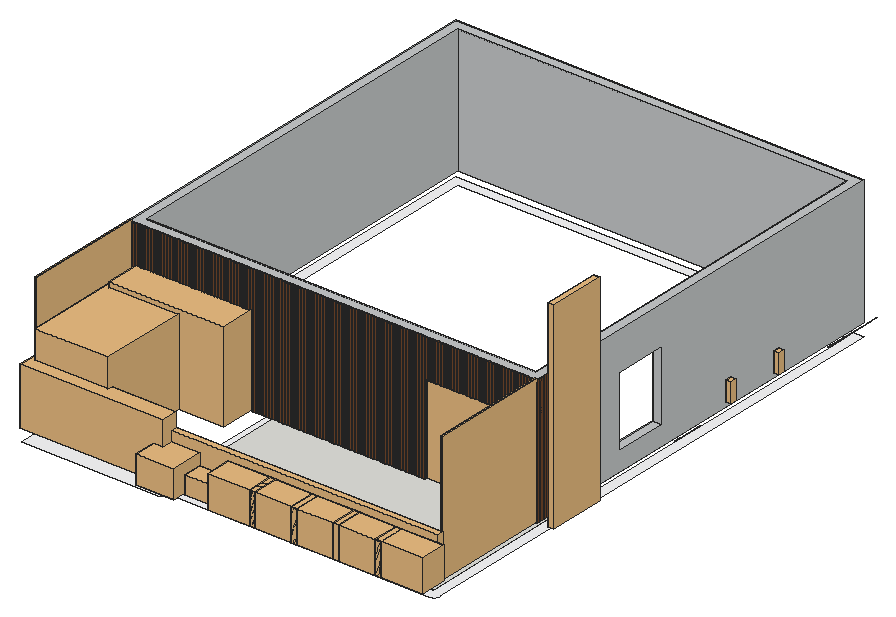
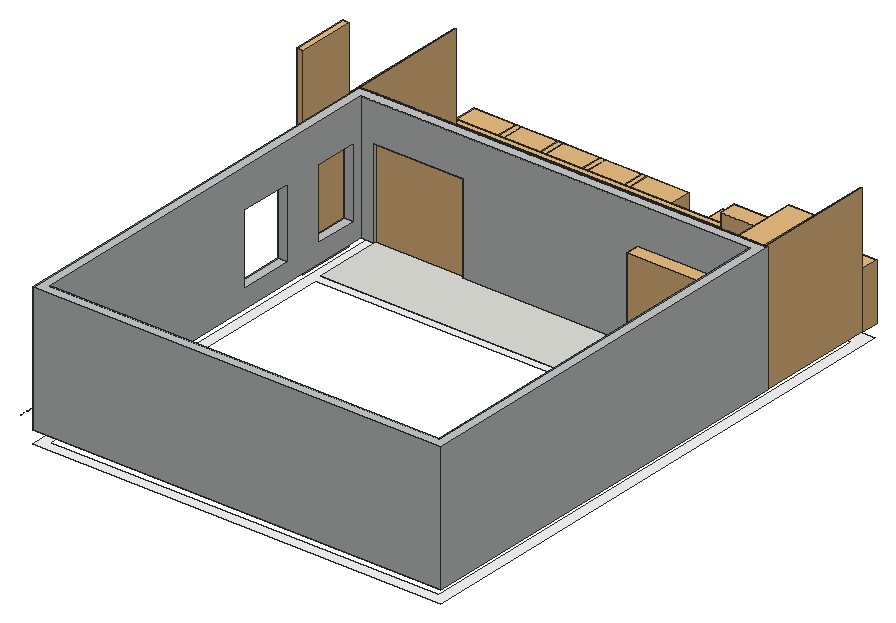
# SketchUp Ruby script. Lengths in inches.
U = 1.inch
M = Sketchup.active_model
def pt(a) = Geom::Point3d.new(a.map { |v| v * U })
def face(e, loops, mat)
  f = e.add_face(loops[0].map { |a| pt(a) })
  loops[1..].each { |l| e.add_face(l.map { |a| pt(a) }).erase! }
  f.material = f.back_material = mat if mat
  f
end
# faces: each face lists its corners as indices into pts; further lists are holes
def faces(e, pts, list, mat = nil) = list.each { |f| face(e, (f[0].is_a?(Array) ? f : [f]).map { |l| l.map { |i| pts[i] } }, mat) }
# xy, xz, yz: faces in a plane at the given z, y or x. An outline is a flat list of corners, or four numbers for a rectangle; further outlines are holes
def ring(l) = l.size == 4 ? [[l[0], l[1]], [l[2], l[1]], [l[2], l[3]], [l[0], l[3]]] : l.each_slice(2).to_a
def flat(e, list, mat, &to3) = list.each { |f| face(e, (f[0].is_a?(Array) ? f : [f]).map { |l| ring(l).map { |u, v| to3.(u, v) } }, mat) }
def xy(e, z, list, mat = nil) = flat(e, list, mat) { |x, y| [x, y, z] }
def xz(e, y, list, mat = nil) = flat(e, list, mat) { |x, z| [x, y, z] }
def yz(e, x, list, mat = nil) = flat(e, list, mat) { |y, z| [x, y, z] }
def lines(e, pts, list) = list.each { |a, b| e.add_line(pt(pts[a]), pt(pts[b])) }
# prism: a flat outline (further loops are holes) pulled along v
def prism(e, loops, v, mat = nil)
  f = face(e, loops, mat); d = Geom::Vector3d.new(v.map { |x| x * U })
  f.pushpull(f.normal.samedirection?(d) ? d.length : -d.length)
end
def box(e, o, s, mat = nil) = prism(e, [[o, [o[0] + s[0], o[1], o[2]], [o[0] + s[0], o[1] + s[1], o[2]], [o[0], o[1] + s[1], o[2]]]], [0, 0, s[2]], mat)
def at(x, y, z, deg = 0) = Geom::Transformation.translation(pt([x, y, z])) * Geom::Transformation.rotation(ORIGIN, Z_AXIS, deg.degrees)
def axes(o, x, y, z) = Geom::Transformation.new([*x, 0, *y, 0, *z, 0, *pt(o).to_a, 1])
def part(name) = M.definitions.add(name)
# library, detail: a bought-in or finely detailed component or shape, given as its bounding box
def library(name, o, s) = part(name).tap { |d| box(d.entities, o, s) }
def detail(e, o, s) = box(e.add_group.entities, o, s)
def put(e, d, t, mat = nil) = e.add_instance(d, t).tap { |i| i.material = mat if mat }
def group(e, t, mat = nil) = e.add_group.tap { |g| g.transformation = t; g.material = mat if mat }.entities
root = M.entities
M.materials.add("1443 AP 8258 WINTER MOON").color = [199, 202, 203]
M.materials.add("[Color G05]").color = [0, 255, 0]
M.materials.add("[Granite Dark Gray]").color = [51, 50, 50]
M.materials.add("[Quartz Light Grey]").color = [251, 251, 252]
M.materials.add("[Wood Cherry Original]").color = [118, 74, 44]
M.materials.add("[Wood Veneer 01]").color = [93, 54, 28]
c1 = part("Group849\#6")
xy(c1.entities,0,[[-15.5,-0.5,15.5,0.5]])
c2 = part("Group849\#1")
xy(c2.entities,0,[[-15.5,-0.5,15.5,0.5]])
c3 = part("Group849\#2")
xy(c3.entities,0,[[-15.5,-0.5,15.5,0.5]])
c4 = library("Group\#13",[0,0,-9],[6,54,189])
c5 = library("123",[7.02,165.98,1.45],[69.08,114.39,80.25])
c6 = library("bi fold",[-79.32,-0.79,-0.5625],[78.74,5.5,90.55])
c7 = library("plants+rack",[-7.12,0,0],[40.64,80.625,63.2])
c8 = library("Group\#7",[-1,-1,-6],[134,16,54])
c9 = part("Group116\#1")
box(c9.entities,[-192,-60,0],[2.5,120,0.5])
c10 = part("Group117\#1")
box(c10.entities,[-189,-60,0],[2.5,120,0.5])
c11 = part("Group118\#1")
box(c11.entities,[-186,-60,0],[2.5,120,0.5])
c12 = part("Group119\#1")
box(c12.entities,[-183,-60,0],[2.5,120,0.5])
c13 = part("Group120\#1")
box(c13.entities,[-180,-60,0],[2.5,120,0.5])
c14 = part("Group121\#1")
box(c14.entities,[-177,-60,0],[2.5,120,0.5])
c15 = part("Group122\#1")
box(c15.entities,[-174,-60,0],[2.5,120,0.5])
c16 = part("Group123\#1")
box(c16.entities,[-171,-60,0],[2.5,120,0.5])
c17 = part("Group124\#1")
box(c17.entities,[-168,-60,0],[2.5,120,0.5])
c18 = part("Group125\#1")
box(c18.entities,[-165,-60,0],[2.5,120,0.5])
c19 = part("Group126\#1")
box(c19.entities,[-162,-60,0],[2.5,120,0.5])
c20 = part("Group127\#1")
box(c20.entities,[-159,-60,0],[2.5,120,0.5])
c21 = part("Group128\#1")
box(c21.entities,[-156,-60,0],[2.5,120,0.5])
c22 = part("Group129\#1")
box(c22.entities,[-153,-60,0],[2.5,120,0.5])
c23 = part("Group130\#1")
box(c23.entities,[-150,-60,0],[2.5,120,0.5])
c24 = part("Group131\#1")
box(c24.entities,[-147,-60,0],[2.5,120,0.5])
c25 = part("Group132\#1")
box(c25.entities,[-144,-60,0],[2.5,120,0.5])
c26 = part("Group133\#1")
box(c26.entities,[-141,-60,0],[2.5,120,0.5])
c27 = part("Group134\#1")
box(c27.entities,[-138,-60,0],[2.5,120,0.5])
c28 = part("Group135\#1")
box(c28.entities,[-135,-60,0],[2.5,120,0.5])
c29 = part("Group136\#1")
box(c29.entities,[-132,-60,0],[2.5,120,0.5])
c30 = part("Group137\#1")
box(c30.entities,[-129,-60,0],[2.5,120,0.5])
c31 = part("Group138\#1")
box(c31.entities,[-126,-60,0],[2.5,120,0.5])
c32 = part("Group139\#1")
box(c32.entities,[-123,-60,0],[2.5,120,0.5])
c33 = part("Group140\#1")
box(c33.entities,[-120,-60,0],[2.5,120,0.5])
c34 = part("Group141\#1")
box(c34.entities,[-117,-60,0],[2.5,120,0.5])
c35 = part("Group142\#1")
box(c35.entities,[-114,-60,0],[2.5,120,0.5])
c36 = part("Group143\#1")
box(c36.entities,[-111,-60,0],[2.5,120,0.5])
c37 = part("Group144\#1")
box(c37.entities,[-108,-60,0],[2.5,120,0.5])
c38 = part("Group145\#1")
box(c38.entities,[-105,-60,0],[2.5,120,0.5])
c39 = part("Group146\#1")
box(c39.entities,[-102,-60,0],[2.5,120,0.5])
c40 = part("Group147\#1")
box(c40.entities,[-99,-60,0],[2.5,120,0.5])
c41 = part("Group148\#1")
box(c41.entities,[-96,-60,0],[2.5,120,0.5])
c42 = part("Group149\#1")
box(c42.entities,[-93,-60,0],[2.5,120,0.5])
c43 = part("Group150\#1")
box(c43.entities,[-90,-60,0],[2.5,120,0.5])
c44 = part("Group151\#1")
box(c44.entities,[-87,-60,0],[2.5,120,0.5])
c45 = part("Group152\#1")
box(c45.entities,[-84,-60,0],[2.5,120,0.5])
c46 = part("Group153\#1")
box(c46.entities,[-81,-60,0],[2.5,120,0.5])
c47 = part("Group154\#1")
box(c47.entities,[-78,-60,0],[2.5,120,0.5])
c48 = part("Group155\#1")
box(c48.entities,[-75,-60,0],[2.5,120,0.5])
c49 = part("Group156\#1")
box(c49.entities,[-72,-60,0],[2.5,120,0.5])
c50 = part("Group157\#1")
box(c50.entities,[-69,-60,0],[2.5,120,0.5])
c51 = part("Group158\#1")
box(c51.entities,[-66,-60,0],[2.5,120,0.5])
c52 = part("Group159\#1")
box(c52.entities,[-63,-60,0],[2.5,120,0.5])
c53 = part("Group160\#1")
box(c53.entities,[-60,-60,0],[2.5,120,0.5])
c54 = part("Group161\#1")
box(c54.entities,[-57,-60,0],[2.5,120,0.5])
c55 = part("Group162\#1")
box(c55.entities,[-54,-60,0],[2.5,120,0.5])
c56 = part("Group163\#1")
box(c56.entities,[-51,-60,0],[2.5,120,0.5])
c57 = part("Group164\#1")
box(c57.entities,[-48,-60,0],[2.5,120,0.5])
c58 = part("Group165\#1")
box(c58.entities,[-45,-60,0],[2.5,120,0.5])
c59 = part("Group166\#1")
box(c59.entities,[-42,-60,0],[2.5,120,0.5])
c60 = part("Group167\#1")
box(c60.entities,[-39,-60,0],[2.5,120,0.5])
c61 = part("Group168\#1")
box(c61.entities,[-36,-60,0],[2.5,120,0.5])
c62 = part("Group169\#1")
box(c62.entities,[-33,-60,0],[2.5,120,0.5])
c63 = part("Group170\#1")
box(c63.entities,[-30,-60,0],[2.5,120,0.5])
c64 = part("Group171\#1")
box(c64.entities,[-27,-60,0],[2.5,120,0.5])
c65 = part("Group172\#1")
box(c65.entities,[-24,-60,0],[2.5,120,0.5])
c66 = part("Group173\#1")
box(c66.entities,[-21,-60,0],[2.5,120,0.5])
c67 = part("Group174\#1")
box(c67.entities,[-18,-60,0],[2.5,120,0.5])
c68 = part("Group175\#1")
box(c68.entities,[-15,-60,0],[2.5,120,0.5])
c69 = part("Group176\#1")
box(c69.entities,[-12,-60,0],[2.5,120,0.5])
c70 = part("Group177\#1")
box(c70.entities,[-9,-60,0],[2.5,120,0.5])
c71 = part("Group178\#1")
box(c71.entities,[-6,-60,0],[2.5,120,0.5])
c72 = part("Group179\#1")
box(c72.entities,[-3,-60,0],[2.5,120,0.5])
c73 = part("Group180\#1")
box(c73.entities,[0,-60,0],[2.5,120,0.5])
c74 = part("Group181\#1")
box(c74.entities,[3,-60,0],[2.5,120,0.5])
c75 = part("Group182\#1")
box(c75.entities,[6,-60,0],[2.5,120,0.5])
c76 = part("Group183\#1")
box(c76.entities,[9,-60,0],[2.5,120,0.5])
c77 = part("Group184\#1")
box(c77.entities,[12,-60,0],[2.5,120,0.5])
c78 = part("Group185\#1")
box(c78.entities,[15,-60,0],[2.5,120,0.5])
c79 = part("Group186\#1")
box(c79.entities,[18,-60,0],[2.5,120,0.5])
c80 = part("Group187\#1")
box(c80.entities,[21,-60,0],[2.5,120,0.5])
c81 = part("Group188\#1")
box(c81.entities,[24,-60,0],[2.5,120,0.5])
c82 = part("Group189\#1")
box(c82.entities,[27,-60,0],[2.5,120,0.5])
c83 = part("Group190\#1")
box(c83.entities,[30,-60,0],[2.5,120,0.5])
c84 = part("Group191\#1")
box(c84.entities,[33,-60,0],[2.5,120,0.5])
c85 = part("Group192\#1")
box(c85.entities,[36,-60,0],[2.5,120,0.5])
c86 = part("Group193\#1")
box(c86.entities,[39,-60,0],[2.5,120,0.5])
c87 = part("Group194\#1")
box(c87.entities,[42,-60,0],[2.5,120,0.5])
c88 = part("Group195\#1")
box(c88.entities,[45,-60,0],[2.5,120,0.5])
c89 = part("Group196\#1")
box(c89.entities,[48,-60,0],[2.5,120,0.5])
c90 = part("Group197\#1")
box(c90.entities,[51,-60,0],[2.5,120,0.5])
c91 = part("Group198\#1")
box(c91.entities,[54,-60,0],[2.5,120,0.5])
c92 = part("Group199\#1")
box(c92.entities,[57,-60,0],[2.5,120,0.5])
c93 = part("Group200\#1")
box(c93.entities,[60,-60,0],[2.5,120,0.5])
c94 = part("Group201\#1")
box(c94.entities,[63,-60,0],[2.5,120,0.5])
c95 = part("Group202\#1")
box(c95.entities,[66,-60,0],[2.5,120,0.5])
c96 = part("Group203\#1")
box(c96.entities,[69,-60,0],[2.5,120,0.5])
c97 = part("Group204\#1")
box(c97.entities,[72,-60,0],[2.5,120,0.5])
c98 = part("Group205\#1")
box(c98.entities,[75,-60,0],[2.5,120,0.5])
c99 = part("Group206\#1")
box(c99.entities,[78,-60,0],[2.5,120,0.5])
c100 = part("Group207\#1")
box(c100.entities,[81,-60,0],[2.5,120,0.5])
c101 = part("Group208\#1")
box(c101.entities,[84,-60,0],[2.5,120,0.5])
c102 = part("Group209\#1")
xy(c102.entities,0,[[87,24,89.5,60]])
xy(c102.entities,0.5,[[87,24,89.5,60]])
xz(c102.entities,60,[[87,0,89.5,0.5]])
yz(c102.entities,87,[[24,0,60,0.5]])
yz(c102.entities,89.5,[[24,0,60,0.5]])
c103 = part("Group210\#1")
box(c103.entities,[90,24,0],[2.5,36,0.5])
c104 = part("Group211\#1")
box(c104.entities,[93,24,0],[2.5,36,0.5])
c105 = part("Group212\#1")
box(c105.entities,[96,24,0],[2.5,36,0.5])
c106 = part("Group213\#1")
box(c106.entities,[99,24,0],[2.5,36,0.5])
c107 = part("Group214\#1")
box(c107.entities,[102,24,0],[2.5,36,0.5])
c108 = part("Group215\#1")
box(c108.entities,[105,24,0],[2.5,36,0.5])
c109 = part("Group216\#1")
box(c109.entities,[108,24,0],[2.5,36,0.5])
c110 = part("Group217\#1")
box(c110.entities,[111,24,0],[2.5,36,0.5])
c111 = part("Group218\#1")
box(c111.entities,[114,24,0],[2.5,36,0.5])
c112 = part("Group219\#1")
box(c112.entities,[117,24,0],[2.5,36,0.5])
c113 = part("Group220\#1")
box(c113.entities,[120,24,0],[2.5,36,0.5])
c114 = part("Group221\#1")
box(c114.entities,[123,24,0],[2.5,36,0.5])
c115 = part("Group222\#1")
box(c115.entities,[126,24,0],[2.5,36,0.5])
c116 = part("Group223\#1")
box(c116.entities,[129,24,0],[2.5,36,0.5])
c117 = part("Group224\#1")
box(c117.entities,[132,24,0],[2.5,36,0.5])
c118 = part("Group225\#1")
box(c118.entities,[135,24,0],[2.5,36,0.5])
c119 = part("Group226\#1")
box(c119.entities,[138,24,0],[2.5,36,0.5])
c120 = part("Group227\#1")
box(c120.entities,[141,24,0],[2.5,36,0.5])
c121 = part("Group228\#1")
box(c121.entities,[144,24,0],[2.5,36,0.5])
c122 = part("Group229\#1")
box(c122.entities,[147,24,0],[2.5,36,0.5])
c123 = part("Group230\#1")
box(c123.entities,[150,24,0],[2.5,36,0.5])
c124 = part("Group231\#1")
box(c124.entities,[153,24,0],[2.5,36,0.5])
c125 = part("Group232\#1")
box(c125.entities,[156,24,0],[2.5,36,0.5])
c126 = part("Group233\#1")
box(c126.entities,[159,24,0],[2.5,36,0.5])
c127 = part("Group234\#1")
box(c127.entities,[162,24,0],[2.5,36,0.5])
c128 = part("Group235\#1")
box(c128.entities,[165,24,0],[2.5,36,0.5])
c129 = part("Group236\#1")
box(c129.entities,[168,24,0],[2.5,36,0.5])
c130 = part("Group237\#1")
prism(c130.entities,[[[173.5,60,0],[173.5,-60,0],[171,-60,0],[171,24,0],[171,60,0]]],[0,0,0.5])
c131 = part("Group238\#1")
box(c131.entities,[174,-60,0],[2.5,120,0.5])
c132 = part("Group239\#1")
box(c132.entities,[177,-60,0],[2.5,120,0.5])
c133 = part("Group240\#1")
box(c133.entities,[180,-60,0],[2.5,120,0.5])
c134 = part("Group241\#1")
box(c134.entities,[183,-60,0],[2.5,120,0.5])
c135 = part("Group242\#1")
box(c135.entities,[186,-60,0],[2.5,120,0.5])
c136 = part("Group243\#1")
box(c136.entities,[189,-60,0],[2.5,120,0.5])
c137 = part("Group114\#1")
put(c137.entities,c9,at(0,0,0))
put(c137.entities,c10,at(0,0,0))
put(c137.entities,c11,at(0,0,0))
put(c137.entities,c12,at(0,0,0))
put(c137.entities,c13,at(0,0,0))
put(c137.entities,c14,at(0,0,0))
put(c137.entities,c15,at(0,0,0))
put(c137.entities,c16,at(0,0,0))
put(c137.entities,c17,at(0,0,0))
put(c137.entities,c18,at(0,0,0))
put(c137.entities,c19,at(0,0,0))
put(c137.entities,c20,at(0,0,0))
put(c137.entities,c21,at(0,0,0))
put(c137.entities,c22,at(0,0,0))
put(c137.entities,c23,at(0,0,0))
put(c137.entities,c24,at(0,0,0))
put(c137.entities,c25,at(0,0,0))
put(c137.entities,c26,at(0,0,0))
put(c137.entities,c27,at(0,0,0))
put(c137.entities,c28,at(0,0,0))
put(c137.entities,c29,at(0,0,0))
put(c137.entities,c30,at(0,0,0))
put(c137.entities,c31,at(0,0,0))
put(c137.entities,c32,at(0,0,0))
put(c137.entities,c33,at(0,0,0))
put(c137.entities,c34,at(0,0,0))
put(c137.entities,c35,at(0,0,0))
put(c137.entities,c36,at(0,0,0))
put(c137.entities,c37,at(0,0,0))
put(c137.entities,c38,at(0,0,0))
put(c137.entities,c39,at(0,0,0))
put(c137.entities,c40,at(0,0,0))
put(c137.entities,c41,at(0,0,0))
put(c137.entities,c42,at(0,0,0))
put(c137.entities,c43,at(0,0,0))
put(c137.entities,c44,at(0,0,0))
put(c137.entities,c45,at(0,0,0))
put(c137.entities,c46,at(0,0,0))
put(c137.entities,c47,at(0,0,0))
put(c137.entities,c48,at(0,0,0))
put(c137.entities,c49,at(0,0,0))
put(c137.entities,c50,at(0,0,0))
put(c137.entities,c51,at(0,0,0))
put(c137.entities,c52,at(0,0,0))
put(c137.entities,c53,at(0,0,0))
put(c137.entities,c54,at(0,0,0))
put(c137.entities,c55,at(0,0,0))
put(c137.entities,c56,at(0,0,0))
put(c137.entities,c57,at(0,0,0))
put(c137.entities,c58,at(0,0,0))
put(c137.entities,c59,at(0,0,0))
put(c137.entities,c60,at(0,0,0))
put(c137.entities,c61,at(0,0,0))
put(c137.entities,c62,at(0,0,0))
put(c137.entities,c63,at(0,0,0))
put(c137.entities,c64,at(0,0,0))
put(c137.entities,c65,at(0,0,0))
put(c137.entities,c66,at(0,0,0))
put(c137.entities,c67,at(0,0,0))
put(c137.entities,c68,at(0,0,0))
put(c137.entities,c69,at(0,0,0))
put(c137.entities,c70,at(0,0,0))
put(c137.entities,c71,at(0,0,0))
put(c137.entities,c72,at(0,0,0))
put(c137.entities,c73,at(0,0,0))
put(c137.entities,c74,at(0,0,0))
put(c137.entities,c75,at(0,0,0))
put(c137.entities,c76,at(0,0,0))
put(c137.entities,c77,at(0,0,0))
put(c137.entities,c78,at(0,0,0))
put(c137.entities,c79,at(0,0,0))
put(c137.entities,c80,at(0,0,0))
put(c137.entities,c81,at(0,0,0))
put(c137.entities,c82,at(0,0,0))
put(c137.entities,c83,at(0,0,0))
put(c137.entities,c84,at(0,0,0))
put(c137.entities,c85,at(0,0,0))
put(c137.entities,c86,at(0,0,0))
put(c137.entities,c87,at(0,0,0))
put(c137.entities,c88,at(0,0,0))
put(c137.entities,c89,at(0,0,0))
put(c137.entities,c90,at(0,0,0))
put(c137.entities,c91,at(0,0,0))
put(c137.entities,c92,at(0,0,0))
put(c137.entities,c93,at(0,0,0))
put(c137.entities,c94,at(0,0,0))
put(c137.entities,c95,at(0,0,0))
put(c137.entities,c96,at(0,0,0))
put(c137.entities,c97,at(0,0,0))
put(c137.entities,c98,at(0,0,0))
put(c137.entities,c99,at(0,0,0))
put(c137.entities,c100,at(0,0,0))
put(c137.entities,c101,at(0,0,0))
put(c137.entities,c102,at(0,0,0))
put(c137.entities,c103,at(0,0,0))
put(c137.entities,c104,at(0,0,0))
put(c137.entities,c105,at(0,0,0))
put(c137.entities,c106,at(0,0,0))
put(c137.entities,c107,at(0,0,0))
put(c137.entities,c108,at(0,0,0))
put(c137.entities,c109,at(0,0,0))
put(c137.entities,c110,at(0,0,0))
put(c137.entities,c111,at(0,0,0))
put(c137.entities,c112,at(0,0,0))
put(c137.entities,c113,at(0,0,0))
put(c137.entities,c114,at(0,0,0))
put(c137.entities,c115,at(0,0,0))
put(c137.entities,c116,at(0,0,0))
put(c137.entities,c117,at(0,0,0))
put(c137.entities,c118,at(0,0,0))
put(c137.entities,c119,at(0,0,0))
put(c137.entities,c120,at(0,0,0))
put(c137.entities,c121,at(0,0,0))
put(c137.entities,c122,at(0,0,0))
put(c137.entities,c123,at(0,0,0))
put(c137.entities,c124,at(0,0,0))
put(c137.entities,c125,at(0,0,0))
put(c137.entities,c126,at(0,0,0))
put(c137.entities,c127,at(0,0,0))
put(c137.entities,c128,at(0,0,0))
put(c137.entities,c129,at(0,0,0))
put(c137.entities,c130,at(0,0,0))
put(c137.entities,c131,at(0,0,0))
put(c137.entities,c132,at(0,0,0))
put(c137.entities,c133,at(0,0,0))
put(c137.entities,c134,at(0,0,0))
put(c137.entities,c135,at(0,0,0))
put(c137.entities,c136,at(0,0,0))
c138 = part("Group376\#1")
box(c138.entities,[-6,-60,0],[1.5,120,0.5])
c139 = part("Group377\#1")
box(c139.entities,[-4,-60,0],[1.5,120,0.5])
c140 = part("Group378\#1")
box(c140.entities,[-2,-60,0],[1.5,120,0.5])
c141 = part("Group379\#1")
box(c141.entities,[0,-60,0],[1.5,120,0.5])
c142 = part("Group380\#1")
box(c142.entities,[2,-60,0],[1.5,120,0.5])
c143 = part("Group381\#1")
box(c143.entities,[4,-60,0],[1.5,120,0.5])
c144 = part("Group374\#2")
put(c144.entities,c138,at(0,0,0))
put(c144.entities,c139,at(0,0,0))
put(c144.entities,c140,at(0,0,0))
put(c144.entities,c141,at(0,0,0))
put(c144.entities,c142,at(0,0,0))
put(c144.entities,c143,at(0,0,0))
c145 = library("23",[0,0,0],[50.58,1.97,105.7])
c146 = library("Group\#23",[0,-49,-2],[251.55,6,45])
c147 = library("Group3_1\#1",[-101.17,21.32,5.81],[18.97,19.56,13.88])
c148 = library("Untitled (9)",[-0.85,-2.66,0],[26.82,17.34,17.35])
c149 = library("ods - 300 x 1000mm Pot Plant",[-1.6,-6.71,0],[44.47,24.63,30.33])
c150 = library("WALL LIGHT 69",[4.19,4.05,-9.63],[4.61,5.7,18.83])
xy(root,256,[[[340.63,149.78,360.41,158.62,360.41,173.83,374.7,180.21,391.73,172.6,411.51,181.4375,411.51,199.11,394.48,206.72,394.48,219.48,411.51,227.08,411.51,244.75,391.73,253.59,374.7,245.98,357.66,253.59,337.88,244.75,337.88,227.08,354.91,219.48,354.91,206.72,337.88,199.11,337.88,183.89,320.85,176.39,320.85,158.62],[340.63,150.6,321.76,159.02,321.76,175.98,338.8,183.48,338.8,198.7,355.83,206.31,355.83,219.88,338.8,227.49,338.8,244.34,357.66,252.77,374.7,245.16,391.73,252.77,410.6,244.34,410.6,227.49,393.5625,219.88,393.5625,206.31,410.6,198.7,410.6,181.85,391.73,173.42,374.7,181.03,359.5,174.24,359.5,159.02]]])
xy(root,257,[[340.63,150.6,359.5,159.02,359.5,174.24,374.7,181.03,391.73,173.42,410.6,181.85,410.6,198.7,393.5625,206.31,393.5625,219.88,410.6,227.49,410.6,244.34,391.73,252.77,374.7,245.16,357.66,252.77,338.8,244.34,338.8,227.49,355.83,219.88,355.83,206.31,338.8,198.7,338.8,183.48,321.76,175.98,321.76,159.02]])
xy(root,258,[[[48,90,174.22,90,174.77,90.05,174.88,90.07,174.99,90.08,175.1,90.1,175.32,90.15,175.43,90.17,175.54,90.2,175.64,90.23,175.75,90.26,175.85,90.29,175.96,90.33,176.0625,90.37,176.17,90.41,176.47,90.53,176.87,90.73,176.97,90.79,177.0625,90.84,177.16,90.9,177.34,91.02,177.4375,91.08,177.53,91.15,177.62,91.21,177.7,91.28,177.79,91.35,177.96,91.49,178.04,91.57,178.125,91.64,178.2,91.72,178.28,91.8,178.36,91.875,178.43,91.96,178.51,92.04,178.65,92.21,178.72,92.3,178.79,92.38,178.85,92.47,178.92,92.5625,178.98,92.66,179.1,92.84,179.16,92.9375,179.21,93.03,179.27,93.13,179.47,93.53,179.59,93.83,179.63,93.9375,179.67,94.04,179.71,94.15,179.74,94.25,179.77,94.36,179.8,94.46,179.83,94.57,179.85,94.68,179.9,94.9,179.92,95.01,179.93,95.12,179.95,95.23,180,95.78,180,96,426.22,96,426.77,96.05,426.88,96.07,426.99,96.08,427.1,96.1,427.32,96.15,427.43,96.17,427.54,96.2,427.64,96.23,427.75,96.26,427.85,96.29,427.96,96.33,428.0625,96.37,428.17,96.41,428.47,96.53,428.87,96.73,428.97,96.79,429.0625,96.84,429.16,96.9,429.34,97.02,429.4375,97.08,429.53,97.15,429.62,97.21,429.7,97.28,429.79,97.35,429.96,97.49,430.04,97.57,430.125,97.64,430.2,97.72,430.28,97.8,430.36,97.875,430.43,97.96,430.51,98.04,430.65,98.21,430.72,98.3,430.79,98.38,430.85,98.47,430.92,98.5625,430.98,98.66,431.1,98.84,431.16,98.9375,431.21,99.03,431.27,99.13,431.47,99.53,431.59,99.83,431.63,99.9375,431.67,100.04,431.71,100.15,431.74,100.25,431.77,100.36,431.8,100.46,431.83,100.57,431.85,100.68,431.9,100.9,431.92,101.01,431.93,101.12,431.95,101.23,432,101.78,432,600,48,600],[57,105,57,591,423,591,423,279,165,279,165,105],[171,105,423,273]]],"[Quartz Light Grey]")
xy(root,259,[[171,105,423,273]])
xy(root,270,[[48,216,48,600,432,600,432,216,411,216,411,225,423,225,423,591,57,591,57,225,327,225,327,216]],"1443 AP 8258 WINTER MOON")
xy(root,278,[[443.875,363,444,369],[443.875,370,444,393],[443.875,543.57,444,591],[443.875,592,444,600]],"[Granite Dark Gray]")
xy(root,288,[[423,234,432,276],[423,312,432,363]],"1443 AP 8258 WINTER MOON")
xy(root,354,[[327,216,411,225],[423,234,432,276],[423,312,432,363]],"1443 AP 8258 WINTER MOON")
xy(root,390,[[[48,216,432,600],[57,225,423,591]]],"1443 AP 8258 WINTER MOON")
xz(root,216,[[48,270,327,270,327,354,411,354,411,270,432,270,432,390,48,390]],"1443 AP 8258 WINTER MOON")
xz(root,225,[[57,270,57,390,423,390,423,270,411,270,411,354,327,354,327,270]],"1443 AP 8258 WINTER MOON")
xz(root,234,[[423,288,432,354]],"1443 AP 8258 WINTER MOON")
xz(root,276,[[423,288,432,354]],"1443 AP 8258 WINTER MOON")
xz(root,312,[[423,288,432,354]],"1443 AP 8258 WINTER MOON")
xz(root,363,[[423,288,432,354]],"1443 AP 8258 WINTER MOON")
xz(root,591,[[57,270,423,390]],"1443 AP 8258 WINTER MOON")
xz(root,600,[[48,270,432,390]],"1443 AP 8258 WINTER MOON")
yz(root,48,[[216,270,600,390]],"1443 AP 8258 WINTER MOON")
yz(root,57,[[225,270,591,390]],"1443 AP 8258 WINTER MOON")
yz(root,320.85,[[158.62,256,176.39,257]],"[Color G05]")
yz(root,327,[[216,270,225,354]],"1443 AP 8258 WINTER MOON")
yz(root,337.88,[[183.89,256,199.11,257],[227.08,256,244.75,257]],"[Color G05]")
yz(root,354.91,[[206.72,256,219.48,257]],"[Color G05]")
yz(root,360.41,[[158.62,256,173.83,257]],"[Color G05]")
yz(root,394.48,[[206.72,256,219.48,257]],"[Color G05]")
yz(root,411,[[216,270,225,354]],"1443 AP 8258 WINTER MOON")
yz(root,411.51,[[181.4375,256,199.11,257],[227.08,256,244.75,257]],"[Color G05]")
yz(root,423,[[[225,270,591,390],[312,288,363,354],[234,288,276,354]]],"1443 AP 8258 WINTER MOON")
yz(root,432,[[216,270,228,390],[[228,270,600,390],[312,288,363,354],[234,288,276,354]]],"1443 AP 8258 WINTER MOON")
p = [[340.63,149.78,257],[320.85,158.62,257],[320.85,158.62,256],[340.63,149.78,256],[360.41,158.62,257],[360.41,158.62,256],
  [391.73,172.6,257],[374.7,180.21,257],[374.7,180.21,256],[391.73,172.6,256],[411.51,181.4375,257],[411.51,181.4375,256],
  [360.41,173.83,257],[360.41,173.83,256],[320.85,176.39,257],[337.88,183.89,257],[337.88,183.89,256],[320.85,176.39,256],
  [337.88,199.11,257],[354.91,206.72,257],[354.91,206.72,256],[337.88,199.11,256],[394.48,206.72,257],[411.51,199.11,257],
  [411.51,199.11,256],[394.48,206.72,256],[354.91,219.48,257],[337.88,227.08,257],[337.88,227.08,256],[354.91,219.48,256],
  [411.51,227.08,257],[394.48,219.48,257],[394.48,219.48,256],[411.51,227.08,256],[337.88,244.75,257],[357.66,253.59,257],
  [357.66,253.59,256],[337.88,244.75,256],[391.73,253.59,257],[411.51,244.75,257],[411.51,244.75,256],[391.73,253.59,256],
  [374.7,245.98,257],[374.7,245.98,256],[196.66,231.6,257],[196.66,214.65,257],[213.69,207.15,257],[213.69,191.93,257],
  [215.52,115.03,257],[232.56,122.64,257],[232.56,262.85,257],[213.69,254.42,257],[268.46,123.46,257],[268.46,138.67,257],
  [230.73,184.32,257],[230.73,169.1,257],[247.76,147.92,257],[232.56,141.13,257],[249.59,115.03,257],[215.52,148.74,257],
  [196.66,140.3125,257],[285.49,146.28,257],[247.76,161.5,257],[285.49,163.13,257],[268.46,170.74,257],[213.69,239.21,257],
  [196.66,123.46,257],[285.49,208.78,257],[266.625,217.21,257],[268.46,184.32,257],[285.49,191.93,257],[249.59,209.6,257],
  [234.39,216.39,257],[234.39,229.97,257],[251.42,237.57,257],[251.42,254.42,257]]
faces(root,p,[[0,1,2,3],[4,0,3,5],[6,7,8,9],[10,6,9,11],[7,12,13,8],[14,15,16,17],[18,19,20,21],[22,23,24,25],
  [26,27,28,29],[30,31,32,33],[34,35,36,37],[38,39,40,41],[35,42,43,36],[42,38,41,43]],"[Color G05]")
lines(root,p,[[44,45],[46,47],[48,49],[50,51],[52,53],[54,55],[56,57],[58,52],[57,59],[59,60],[45,46],[49,58],
  [47,54],[53,61],[62,56],[63,64],[51,65],[55,62],[60,66],[67,68],[69,70],[68,71],[72,73],[64,69],
  [61,63],[73,74],[71,72],[70,67],[74,75],[75,50],[66,48]])
put(root,c1,axes([243.82,233.36,256.5],[-0.54948,-0.2454,0],[0,0,1],[0.45818,-0.61389,0]))
put(root,c1,axes([277.89,187.71,256.5],[-0.54948,-0.2454,0],[0,0,1],[0.45818,-0.61389,0]))
put(root,c1,axes([277.89,142.07,256.5],[-0.54948,-0.2454,0],[0,0,1],[0.45818,-0.61389,0]))
put(root,c1,axes([259.48,118.63,256.5],[-0.63816,-0.28501,0],[0,0,1],[0.45818,-0.61389,0]))
put(root,c1,axes([224.04,118.02,256.5],[-0.54948,-0.2454,0],[0,0,1],[0.45818,-0.61389,0]))
put(root,c1,axes([252.34,246,256.5],[0,-0.57002,0],[0,0,1],[0.91636,0,0]))
put(root,c1,axes([235.31,223.21,256.5],[0,-0.40952,0],[0,0,1],[0.91636,0,0]))
put(root,c1,axes([286.41,200.35,256.5],[0,-0.57002,0],[0,0,1],[0.91636,0,0]))
put(root,c1,axes([286.41,154.71,256.5],[0,-0.57002,0],[0,0,1],[0.91636,0,0]))
put(root,c2,axes([269.375,130.66,256.5],[0,-0.49081,0],[0,0,1],[0.91636,0,0]))
put(root,c1,axes([204.26,235.82,256.5],[0.54948,0.2454,0],[0,0,-1],[-0.45818,0.61389,0]))
put(root,c1,axes([212.78,199.125,256.5],[0,0.49081,0],[0,0,-1],[-0.91636,0,0]))
put(root,c1,axes([195.74,224.4,256.5],[0,0.49081,0],[0,0,-1],[-0.91636,0,0]))
put(root,c1,axes([229.81,176.3,256.5],[0,0.49081,0],[0,0,-1],[-0.91636,0,0]))
put(root,c1,axes([246.84,154.7,256.5],[0,0.41228,0],[0,0,-1],[-0.91636,0,0]))
put(root,c1,axes([195.74,133.11,256.5],[0,0.49081,0],[0,0,-1],[-0.91636,0,0]))
put(root,c1,axes([242.45,259.25,256.5],[0.63816,-0.28501,0],[0,0,-1],[0.45818,0.61389,0]))
put(root,c3,axes([277.89,167.35,256.5],[0.54948,-0.2454,0],[0,0,-1],[0.45818,0.61389,0]))
put(root,c1,axes([224.04,145.75,256.5],[0.54948,-0.2454,0],[0,0,-1],[0.45818,0.61389,0]))
put(root,c1,axes([242.45,213.61,256.5],[0.4608,-0.2058,0],[0,0,-1],[0.45818,0.61389,0]))
put(root,c1,axes([239.7,145.14,256.5],[0.4608,0.2058,0],[0,0,-1],[-0.45818,0.61389,0]))
put(root,c1,axes([222.7,259.29,256.5],[0.6359,0.284,0],[0,0,-1],[-0.45818,0.61389,0]))
put(root,c1,axes([222.67,187.1,256.5],[-0.4608,0.2058,0],[0,0,-1],[-0.45818,-0.61389,0]))
put(root,c1,axes([208.38,117.41,256.5],[-0.4608,0.2058,0],[0,0,-1],[-0.45818,-0.61389,0]))
put(root,c1,axes([241.09,118.01,256.5],[-0.54835,0.2449,0],[0,0,-1],[-0.45818,-0.61389,0]))
put(root,c1,axes([330.74,154.2,256.5],[-0.63816,0.28501,0],[0,0,-1],[-0.45818,-0.61389,0]))
put(root,c1,axes([383.21,176.41,256.5],[-0.54948,0.2454,0],[0,0,-1],[-0.45818,-0.61389,0]))
put(root,c1,axes([401.62,177.02,256.5],[-0.63816,-0.28501,0],[0,0,-1],[0.45818,-0.61389,0]))
put(root,c1,axes([411.51,190.27,256.5],[0,-0.57002,0],[0,0,-1],[0.91636,0,0]))
put(root,c1,axes([394.48,213.09,256.5],[0,-0.41205,0],[0,0,-1],[0.91636,0,0]))
put(root,c1,axes([411.51,235.92,256.5],[0,-0.57002,0],[0,0,-1],[0.91636,0,0]))
put(root,c1,axes([360.41,166.22,256.5],[0,-0.49081,0],[0,0,-1],[0.91636,0,0]))
put(root,c1,axes([367.55,177.02,256.5],[-0.4608,-0.2058,0],[0,0,-1],[0.45818,-0.61389,0]))
put(root,c1,axes([350.52,154.2,256.5],[-0.63816,-0.28501,0],[0,0,-1],[0.45818,-0.61389,0]))
put(root,c1,axes([403,223.28,256.5],[-0.54948,-0.2454,0],[0,0,-1],[0.45818,-0.61389,0]))
put(root,c1,axes([402.98,202.92,256.5],[0.54835,-0.2449,0],[0,0,-1],[0.45818,0.61389,0]))
put(root,c1,axes([398.87,250.4,256.5],[0.4608,-0.2058,0],[0,0,-1],[0.45818,0.61389,0]))
put(root,c1,axes([364.81,250.4,256.5],[0.4608,-0.2058,0],[0,0,-1],[0.45818,0.61389,0]))
put(root,c1,axes([273.77,214.83,256.5],[0.4608,-0.2058,0],[0,0,-1],[0.45818,0.61389,0]))
put(root,c1,axes([239.7,260.48,256.5],[0.4608,-0.2058,0],[0,0,-1],[0.45818,0.61389,0]))
put(root,c1,axes([347.77,249.17,256.5],[0.63816,0.28501,0],[0,0,-1],[-0.45818,0.61389,0]))
put(root,c1,axes([346.4,202.91,256.5],[0.54948,0.2454,0],[0,0,-1],[-0.45818,0.61389,0]))
put(root,c1,axes([329.36,180.09,256.5],[0.54948,0.2454,0],[0,0,-1],[-0.45818,0.61389,0]))
put(root,c1,axes([383.21,249.79,256.5],[0.54948,0.2454,0],[0,0,-1],[-0.45818,0.61389,0]))
put(root,c1,axes([354.91,213.1,256.5],[0,0.4116,0],[0,0,-1],[-0.91636,0,0]))
put(root,c1,axes([337.88,191.5,256.5],[0,0.49081,0],[0,0,-1],[-0.91636,0,0]))
put(root,c1,axes([320.85,167.44,256.5],[0,0.56934,0],[0,0,-1],[-0.91636,0,0]))
put(root,c1,axes([346.34,223.3,256.5],[-0.55296,0.24696,0],[0,0,-1],[-0.45818,-0.61389,0]))
put(root,c1,axes([212.78,247.23,256.5],[0,0.49081,0],[0,0,-1],[-0.91636,0,0]))
put(root,c1,axes([337.88,234.69,256.5],[0,0.49081,0],[0,0,-1],[-0.91636,0,0]))
put(root,c1,axes([207.01,145.75,256.5],[0.54948,0.2454,0],[0,0,-1],[-0.45818,0.61389,0]))
put(root,c1,axes([239.7,164.28,256.5],[-0.4608,0.2058,0],[0,0,-1],[-0.45818,-0.61389,0]))
put(root,c1,axes([205.63,209.92,256.5],[-0.4608,0.2058,0],[0,0,-1],[-0.45818,-0.61389,0]))
put(root,c1,axes([269.375,177.5625,256.5],[0,-0.40952,0],[0,0,1],[0.91636,0,0]))
put(root,c1,axes([258.08,214.24,256.56],[0.54723,0.24638,0.00361],[0.00424,0.00174,-0.99999],[-0.46095,0.61265,-0.00021]))
put(root,c1,axes([221.26,258.65,256.56],[0.54723,0.24638,0.00361],[0.00424,0.00174,-0.99999],[-0.46095,0.61265,-0.00021]))
put(root,c4,at(432,228,270),"[Quartz Light Grey]")
put(root,c5,at(43.98,-64.87,268.51))
put(root,c6,axes([411.62,218.29,270.52],[1.0668,0,0],[0,1,0],[0,0,0.92765]),"[Quartz Light Grey]")
put(root,c7,axes([54.88,228.6875,270],[0,-1.34,0],[1.34,0,0],[0,0,1.34]))
put(root,c8,at(48,90,276),"[Quartz Light Grey]")
g1 = group(root,at(48,216,270),"[Wood Cherry Original]")
put(g1,c137,axes([192,0,60],[1,0,0],[0,0,1],[0,-1,0]))
g2 = group(root,at(432,216,270),"[Wood Cherry Original]")
put(g2,c144,axes([0,6,60],[0,1,0],[0,0,1],[1,0,0]))
put(root,c145,axes([431.82,105,270],[0,2.19434,0],[-1,0,0],[0,0,1.14472]))
put(root,c145,axes([48.18,105,270],[0,2.19434,0],[1,0,0],[0,0,1.14472]))
put(root,c146,axes([180,148,271.82],[1.003,0,0],[0,1,0],[0,0,0.91111]),"[Wood Veneer 01]")
put(root,c147,axes([362.78,28.39,264.62],[1.88,0,0],[0,1.88,0],[0,0,1.88]))
put(root,c148,at(211.75,80.66,276))
put(root,c149,at(238.84,78,276))
put(root,c149,at(278.34,78,276))
put(root,c149,at(317.84,78,276))
put(root,c149,at(357.34,78,276))
put(root,c149,at(396.84,78,276))
put(root,c150,at(432.81,428.03,288.01))
put(root,c150,at(432.81,483.93,288.01))
